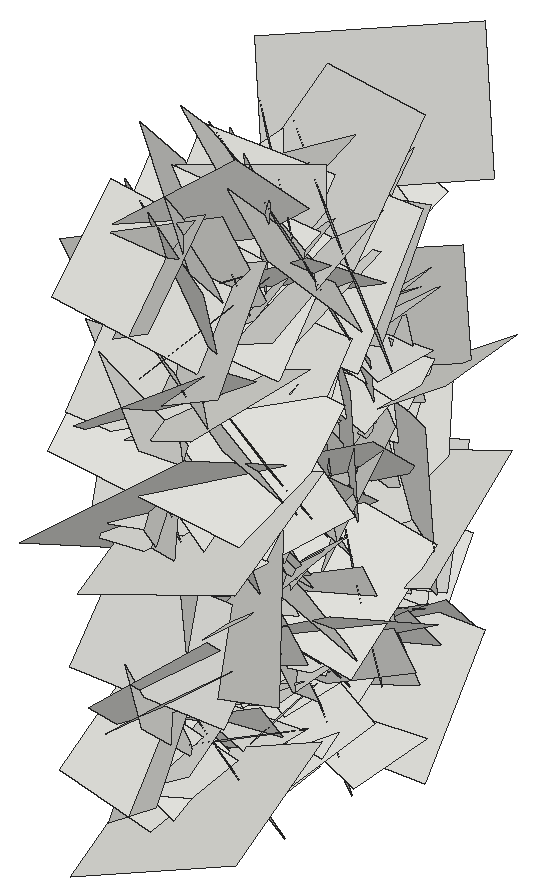
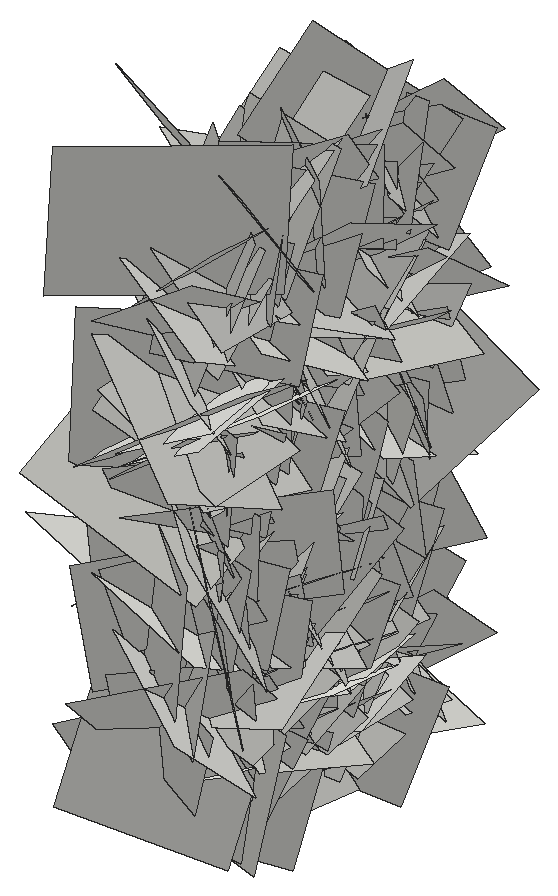
# SketchUp Ruby script. Lengths in inches.
U = 1.inch
M = Sketchup.active_model
def pt(a) = Geom::Point3d.new(a.map { |v| v * U })
def face(e, loops, mat)
  f = e.add_face(loops[0].map { |a| pt(a) })
  loops[1..].each { |l| e.add_face(l.map { |a| pt(a) }).erase! }
  f.material = f.back_material = mat if mat
  f
end
# faces: each face lists its corners as indices into pts; further lists are holes
def faces(e, pts, list, mat = nil) = list.each { |f| face(e, (f[0].is_a?(Array) ? f : [f]).map { |l| l.map { |i| pts[i] } }, mat) }
# xy, xz, yz: faces in a plane at the given z, y or x. An outline is a flat list of corners, or four numbers for a rectangle; further outlines are holes
def ring(l) = l.size == 4 ? [[l[0], l[1]], [l[2], l[1]], [l[2], l[3]], [l[0], l[3]]] : l.each_slice(2).to_a
def flat(e, list, mat, &to3) = list.each { |f| face(e, (f[0].is_a?(Array) ? f : [f]).map { |l| ring(l).map { |u, v| to3.(u, v) } }, mat) }
def xy(e, z, list, mat = nil) = flat(e, list, mat) { |x, y| [x, y, z] }
def xz(e, y, list, mat = nil) = flat(e, list, mat) { |x, z| [x, y, z] }
def yz(e, x, list, mat = nil) = flat(e, list, mat) { |y, z| [x, y, z] }
def lines(e, pts, list) = list.each { |a, b| e.add_line(pt(pts[a]), pt(pts[b])) }
# prism: a flat outline (further loops are holes) pulled along v
def prism(e, loops, v, mat = nil)
  f = face(e, loops, mat); d = Geom::Vector3d.new(v.map { |x| x * U })
  f.pushpull(f.normal.samedirection?(d) ? d.length : -d.length)
end
def box(e, o, s, mat = nil) = prism(e, [[o, [o[0] + s[0], o[1], o[2]], [o[0] + s[0], o[1] + s[1], o[2]], [o[0], o[1] + s[1], o[2]]]], [0, 0, s[2]], mat)
def at(x, y, z, deg = 0) = Geom::Transformation.translation(pt([x, y, z])) * Geom::Transformation.rotation(ORIGIN, Z_AXIS, deg.degrees)
def axes(o, x, y, z) = Geom::Transformation.new([*x, 0, *y, 0, *z, 0, *pt(o).to_a, 1])
def part(name) = M.definitions.add(name)
# library, detail: a bought-in or finely detailed component or shape, given as its bounding box
def library(name, o, s) = part(name).tap { |d| box(d.entities, o, s) }
def detail(e, o, s) = box(e.add_group.entities, o, s)
def put(e, d, t, mat = nil) = e.add_instance(d, t).tap { |i| i.material = mat if mat }
def group(e, t, mat = nil) = e.add_group.tap { |g| g.transformation = t; g.material = mat if mat }.entities
root = M.entities
c1 = part("Component\#6")
p = [[0.01,0,0],[0,3.24,4.54],[4.32,3.24,4.54],[4.33,0,0]]
faces(c1.entities,p,[[0,1,2,3]])
put(root,c1,axes([38.11,167.01,8.33],[-0.18631,0.3359,0.73427],[-0.04897,0.74605,-0.35235],[-0.8545,-0.11599,-0.1399]))
put(root,c1,axes([34.14,159.82,10.86],[-0.164,0.05549,-0.7166],[0.119,-0.72215,-0.08015],[0.75252,0.12629,-0.14349]))
put(root,c1,axes([38.11,164.72,6.23],[0.02586,0.29335,1.1723],[0.23754,1.1511,-0.29271],[-1.25874,0.22326,-0.03115]))
put(root,c1,axes([34.14,164.71,11.17],[-0.09162,-0.23701,0.75882],[-0.09076,0.76162,0.22813],[0.83777,0.05659,0.1077]))
put(root,c1,axes([34.14,167.39,12.19],[-0.06725,0.11282,-0.6237],[0.12717,-0.61335,-0.12315],[0.65971,0.12973,-0.03984]))
put(root,c1,axes([34.14,158.25,7.85],[0.01053,0.60228,-0.51533],[-0.19634,-0.49934,-0.58716],[0.81696,-0.12777,-0.13447]))
put(root,c1,axes([38.11,165.51,17.74],[-0.00528,-0.97827,-0.44464],[0.11526,-0.44282,0.97306],[-1.13321,-0.04048,0.10104]))
put(root,c1,axes([38.11,165.75,-1.09],[0.03685,-0.4153,0.96157],[0.02645,0.96216,0.41465],[-1.10996,0.00914,0.04181]))
put(root,c1,axes([38.11,167.74,3.51],[0.11337,-0.86322,0.3774],[-0.28126,0.33685,0.84566],[-0.95821,-0.201,-0.20357]))
put(root,c1,axes([38.11,161.03,4.22],[-0.00206,0.54706,-0.73945],[-0.10036,-0.73565,-0.544],[-0.96983,0.07497,0.05787]))
put(root,c1,axes([38.11,158.84,13.7],[-0.15038,-0.75335,0.50607],[0.08727,0.49942,0.76653],[-0.95804,0.16374,-0.00961]))
put(root,c1,axes([38.11,166.72,20.27],[-0.14718,0.45385,-0.66356],[-0.05291,-0.67695,-0.45256],[-0.85051,-0.03642,0.14299]))
put(root,c1,axes([34.14,158.82,19.64],[0.09205,0.73549,-0.019],[-0.17536,0.00088,-0.72213],[0.75991,-0.08889,-0.16434]))
put(root,c1,axes([38.11,169.09,13.37],[-0.12805,-0.81492,0.2825],[0.01832,0.28292,0.8235],[-0.91406,0.11983,-0.02307]))
put(root,c1,axes([34.14,159.61,12.59],[0.0897,0.16152,-0.57424],[0.01993,-0.58042,-0.16049],[0.632,-0.00462,0.08656]))
put(root,c1,axes([34.14,160.65,18.69],[0.1336,-0.1743,0.59472],[-0.06624,0.60023,0.18916],[0.65357,0.09646,-0.1024]))
put(root,c1,axes([34.14,160.54,14.42],[-0.065,-0.29459,-0.75204],[-0.0763,-0.74921,0.29935],[0.85274,-0.0895,-0.03054]))
put(root,c1,axes([34.14,161.26,10.83],[-0.08958,0.45503,-0.59155],[0.06652,-0.58889,-0.46195],[0.78829,0.10141,-0.02824]))
put(root,c1,axes([38.11,170.16,13.55],[0.14984,-1.04824,-0.22204],[-0.00627,-0.22472,1.05715],[-1.13577,-0.13705,-0.03513]))
put(root,c1,axes([34.14,160.97,6.7],[0.04912,0.73058,0.10133],[-0.09877,0.10652,-0.72536],[0.77557,-0.03271,-0.0988]))
put(root,c1,axes([38.11,163.26,10.51],[-0.09772,0.8385,-0.3881],[0.10419,-0.37892,-0.842],[-0.97385,-0.12468,-0.05114]))
put(root,c1,axes([34.14,159.79,25.07],[-0.1328,0.69586,-0.68383],[-0.18687,-0.69425,-0.67416],[1.01714,-0.03669,-0.21313]))
put(root,c1,axes([38.11,167.39,3.05],[0.22625,-1.02118,-0.283],[-0.12014,-0.30902,1.02962],[-1.11681,-0.17363,-0.16809]))
put(root,c1,axes([34.14,159.32,12.84],[0.06752,-0.16321,-0.59207],[0.0871,-0.58763,0.17083],[0.64514,0.09641,0.0389]))
put(root,c1,axes([34.14,169.73,5.36],[0.07377,0.11031,-0.61615],[0.06228,-0.61836,-0.10407],[0.66058,0.04598,0.07863]))
put(root,c1,axes([38.11,166.22,16.78],[0.0558,0.90138,-0.08554],[-0.09664,-0.07998,-0.89882],[-0.95488,0.06076,0.08597]))
put(root,c1,axes([34.14,166.8,6.58],[-0.19077,-0.84984,-0.315],[0.00737,-0.32244,0.86593],[0.9607,-0.16629,-0.0692]))
put(root,c1,axes([38.11,159.03,23.29],[0.13252,0.38295,-0.87838],[-0.10893,-0.87536,-0.39626],[-1.00987,0.14467,-0.07253]))
put(root,c1,axes([34.14,160.57,3.12],[0.03509,0.82869,0.13415],[-0.15764,0.13792,-0.81528],[0.87577,-0.00838,-0.15213]))
put(root,c1,axes([34.14,164.04,15.7],[0.03624,-0.6234,-0.24842],[0.08,-0.24359,0.62167],[0.70683,0.05954,-0.05762]))
put(root,c1,axes([38.11,170.98,12.21],[0.31631,-0.51758,-1.19288],[0.16648,-1.20059,0.56021],[-1.36826,-0.26573,-0.20761]))
put(root,c1,axes([34.14,169.83,13.22],[0.13817,-0.64015,-0.16037],[-0.03989,-0.17041,0.64965],[0.69839,0.11692,0.06883]))
put(root,c1,axes([34.14,161.46,7.67],[0.11157,-0.00104,0.59962],[0.09459,0.60203,-0.01462],[0.62852,-0.09042,-0.10424]))
put(root,c1,axes([38.11,168.08,9.41],[0.11593,0.02752,-0.90523],[-0.14705,-0.90054,-0.04413],[-0.94866,0.14295,-0.10378]))
put(root,c1,axes([34.14,169.26,18.83],[0.02849,-0.83115,-0.05333],[-0.13283,-0.05679,0.82186],[0.87278,0.01849,0.12683]))
put(root,c1,axes([34.14,165.55,15.88],[-0.02597,-0.35934,-0.67832],[0.02345,-0.67872,0.35875],[0.81334,0.00809,-0.032]))
put(root,c1,axes([34.14,167.12,21.5],[0.0656,0.35319,-0.61189],[0.00255,-0.61434,-0.35436],[0.7489,-0.02885,0.0548]))
put(root,c1,axes([38.11,164.04,2.37],[0.08884,-0.86849,0.07962],[-0.14736,0.06566,0.86256],[-0.91264,-0.09515,-0.13152]))
put(root,c1,axes([38.11,162.54,0.74],[0.05881,-0.79857,0.25436],[-0.14334,0.24305,0.79255],[-0.87675,-0.0933,-0.11251]))
put(root,c1,axes([38.11,157.37,3.29],[-0.12325,0.67494,0.21472],[-0.06797,0.20667,-0.68436],[-0.74769,-0.13004,0.02682]))
put(root,c1,axes([38.11,166.02,4.84],[0.16866,0.71959,0.68076],[-0.0323,0.69272,-0.72511],[-1.04952,0.09433,0.13172]))
put(root,c1,axes([34.14,162.4,12.14],[0.15913,-0.1111,0.71617],[-0.10617,0.72117,0.13287],[0.76084,0.12387,-0.13124]))
put(root,c1,axes([34.14,165.06,16.01],[-0.24936,0.99659,0.4051],[-0.07669,0.39908,-1.02378],[1.13774,0.24532,0.01978]))
put(root,c1,axes([34.14,164.7,6.68],[-0.19863,-0.78204,0.62344],[-0.03401,0.63866,0.7915],[1.0596,-0.1261,0.14227]))
put(root,c1,axes([38.11,166.67,11.65],[-0.03639,0.32382,0.70516],[-0.0632,0.70266,-0.32558],[-0.82009,-0.06852,-0.0062]))
put(root,c1,axes([38.11,166.25,3.34],[-0.10377,-0.78092,-0.09398],[0.04515,-0.09983,0.78516],[-0.83253,0.09192,0.05429]))
put(root,c1,axes([38.11,167.84,10.46],[0.01526,0.23241,-0.73689],[-0.14958,-0.72384,-0.23105],[-0.80526,0.13886,0.02896]))
put(root,c1,axes([38.11,164.66,7.18],[0.03191,0.54978,-0.59147],[-0.106,-0.58478,-0.54866],[-0.84939,0.09364,0.04625]))
put(root,c1,axes([38.11,155.24,20.59],[-0.01301,0.69003,0.71111],[0.211,0.69839,-0.67424],[-1.02891,0.13449,-0.14726]))
put(root,c1,axes([38.11,167.39,19.82],[-0.12929,0.6108,0.35138],[-0.02449,0.35295,-0.62154],[-0.74654,-0.11736,-0.04046]))
put(root,c1,axes([34.14,165.07,9.38],[0.13081,0.27606,-0.70722],[-0.08788,-0.70731,-0.29057],[0.79993,-0.12284,0.08373]))
put(root,c1,axes([38.11,159.79,6],[0.13547,0.51146,0.93772],[0.15367,0.92736,-0.52557],[-1.12174,0.18881,0.04125]))
put(root,c1,axes([38.11,159.9,13.67],[0.02397,0.44215,0.82689],[0.11898,0.8199,-0.44149],[-0.98679,0.1096,-0.03314]))
put(root,c1,axes([34.14,164.44,22.83],[-0.02931,-0.02413,-0.88007],[-0.04764,-0.87932,0.02552],[0.93201,-0.0457,-0.02637]))
put(root,c1,axes([38.11,168.54,15.47],[0.051,0.16682,-0.79913],[-0.09039,-0.79511,-0.17112],[-0.86061,0.0934,-0.02938]))
put(root,c1,axes([38.11,155.625,2.89],[-0.13104,0.56412,0.5606],[0.11872,0.57403,-0.55293],[-0.83462,-0.00692,-0.16667]))
put(root,c1,axes([38.11,163.43,17.5],[0.07736,-0.30856,0.98844],[0.18729,0.98007,0.2929],[-1.08152,0.14765,0.12143]))
put(root,c1,axes([34.14,163.43,17.5],[-0.07736,-0.30856,0.98844],[-0.18729,0.98007,0.2929],[1.08152,0.14765,0.12143]))
put(root,c1,axes([34.14,155.625,2.89],[0.13104,0.56412,0.5606],[-0.11872,0.57403,-0.55293],[0.83462,-0.00692,-0.16667]))
put(root,c1,axes([34.14,168.54,15.47],[-0.051,0.16682,-0.79913],[0.09039,-0.79511,-0.17112],[0.86061,0.0934,-0.02938]))
put(root,c1,axes([38.11,164.44,22.83],[0.02931,-0.02413,-0.88007],[0.04764,-0.87932,0.02552],[-0.93201,-0.0457,-0.02637]))
put(root,c1,axes([34.14,159.9,13.67],[-0.02397,0.44215,0.82689],[-0.11898,0.8199,-0.44149],[0.98679,0.1096,-0.03314]))
put(root,c1,axes([34.14,159.79,6],[-0.13547,0.51146,0.93772],[-0.15367,0.92736,-0.52557],[1.12174,0.18881,0.04125]))
put(root,c1,axes([38.11,165.07,9.38],[-0.13081,0.27606,-0.70722],[0.08788,-0.70731,-0.29057],[-0.79993,-0.12284,0.08373]))
put(root,c1,axes([34.14,167.39,19.82],[0.12929,0.6108,0.35138],[0.02449,0.35295,-0.62154],[0.74654,-0.11736,-0.04046]))
put(root,c1,axes([34.14,155.24,20.59],[0.01301,0.69003,0.71111],[-0.211,0.69839,-0.67424],[1.02891,0.13449,-0.14726]))
put(root,c1,axes([34.14,164.66,7.18],[-0.03191,0.54978,-0.59147],[0.106,-0.58478,-0.54866],[0.84939,0.09364,0.04625]))
put(root,c1,axes([34.14,167.84,10.46],[-0.01526,0.23241,-0.73689],[0.14958,-0.72384,-0.23105],[0.80526,0.13886,0.02896]))
put(root,c1,axes([34.14,166.25,3.34],[0.10377,-0.78092,-0.09398],[-0.04515,-0.09983,0.78516],[0.83253,0.09192,0.05429]))
put(root,c1,axes([34.14,166.67,11.65],[0.03639,0.32382,0.70516],[0.0632,0.70266,-0.32558],[0.82009,-0.06852,-0.0062]))
put(root,c1,axes([38.11,164.7,6.68],[0.19863,-0.78204,0.62344],[0.03401,0.63866,0.7915],[-1.0596,-0.1261,0.14227]))
put(root,c1,axes([38.11,165.06,16.01],[0.24936,0.99659,0.4051],[0.07669,0.39908,-1.02378],[-1.13774,0.24532,0.01978]))
put(root,c1,axes([38.11,162.4,12.14],[-0.15913,-0.1111,0.71617],[0.10617,0.72117,0.13287],[-0.76084,0.12387,-0.13124]))
put(root,c1,axes([34.14,166.02,4.84],[-0.16866,0.71959,0.68076],[0.0323,0.69272,-0.72511],[1.04952,0.09433,0.13172]))
put(root,c1,axes([34.14,157.37,3.29],[0.12325,0.67494,0.21472],[0.06797,0.20667,-0.68436],[0.74769,-0.13004,0.02682]))
put(root,c1,axes([34.14,162.54,0.74],[-0.05881,-0.79857,0.25436],[0.14334,0.24305,0.79255],[0.87675,-0.0933,-0.11251]))
put(root,c1,axes([34.14,164.04,2.37],[-0.08884,-0.86849,0.07962],[0.14736,0.06566,0.86256],[0.91264,-0.09515,-0.13152]))
put(root,c1,axes([38.11,167.12,21.5],[-0.0656,0.35319,-0.61189],[-0.00255,-0.61434,-0.35436],[-0.7489,-0.02885,0.0548]))
put(root,c1,axes([38.11,165.55,15.88],[0.02597,-0.35934,-0.67832],[-0.02345,-0.67872,0.35875],[-0.81334,0.00809,-0.032]))
put(root,c1,axes([38.11,169.26,18.83],[-0.02849,-0.83115,-0.05333],[0.13283,-0.05679,0.82186],[-0.87278,0.01849,0.12683]))
put(root,c1,axes([34.14,168.08,9.41],[-0.11593,0.02752,-0.90523],[0.14705,-0.90054,-0.04413],[0.94866,0.14295,-0.10378]))
put(root,c1,axes([38.11,161.46,7.67],[-0.11157,-0.00104,0.59962],[-0.09459,0.60203,-0.01462],[-0.62852,-0.09042,-0.10424]))
put(root,c1,axes([38.11,169.83,13.22],[-0.13817,-0.64015,-0.16037],[0.03989,-0.17041,0.64965],[-0.69839,0.11692,0.06883]))
put(root,c1,axes([34.14,170.98,12.21],[-0.31631,-0.51758,-1.19288],[-0.16648,-1.20059,0.56021],[1.36826,-0.26573,-0.20761]))
put(root,c1,axes([38.11,164.04,15.7],[-0.03624,-0.6234,-0.24842],[-0.08,-0.24359,0.62167],[-0.70683,0.05954,-0.05762]))
put(root,c1,axes([38.11,160.57,3.12],[-0.03509,0.82869,0.13415],[0.15764,0.13792,-0.81528],[-0.87577,-0.00838,-0.15213]))
put(root,c1,axes([34.14,159.03,23.29],[-0.13252,0.38295,-0.87838],[0.10893,-0.87536,-0.39626],[1.00987,0.14467,-0.07253]))
put(root,c1,axes([38.11,166.8,6.58],[0.19077,-0.84984,-0.315],[-0.00737,-0.32244,0.86593],[-0.9607,-0.16629,-0.0692]))
put(root,c1,axes([34.14,166.22,16.78],[-0.0558,0.90138,-0.08554],[0.09664,-0.07998,-0.89882],[0.95488,0.06076,0.08597]))
put(root,c1,axes([38.11,159.32,12.84],[-0.06752,-0.16321,-0.59207],[-0.0871,-0.58763,0.17083],[-0.64514,0.09641,0.0389]))
put(root,c1,axes([34.14,167.39,3.05],[-0.22625,-1.02118,-0.283],[0.12014,-0.30902,1.02962],[1.11681,-0.17363,-0.16809]))
put(root,c1,axes([38.11,159.79,25.07],[0.1328,0.69586,-0.68383],[0.18687,-0.69425,-0.67416],[-1.01714,-0.03669,-0.21313]))
put(root,c1,axes([34.14,163.26,10.51],[0.09772,0.8385,-0.3881],[-0.10419,-0.37892,-0.842],[0.97385,-0.12468,-0.05114]))
put(root,c1,axes([38.11,160.97,6.7],[-0.04912,0.73058,0.10133],[0.09877,0.10652,-0.72536],[-0.77557,-0.03271,-0.0988]))
put(root,c1,axes([34.14,170.16,13.55],[-0.14984,-1.04824,-0.22204],[0.00627,-0.22472,1.05715],[1.13577,-0.13705,-0.03513]))
put(root,c1,axes([38.11,161.26,10.83],[0.08958,0.45503,-0.59155],[-0.06652,-0.58889,-0.46195],[-0.78829,0.10141,-0.02824]))
put(root,c1,axes([38.11,160.54,14.42],[0.065,-0.29459,-0.75204],[0.0763,-0.74921,0.29935],[-0.85274,-0.0895,-0.03054]))
put(root,c1,axes([38.11,160.65,18.69],[-0.1336,-0.1743,0.59472],[0.06624,0.60023,0.18916],[-0.65357,0.09646,-0.1024]))
put(root,c1,axes([38.11,159.61,12.59],[-0.0897,0.16152,-0.57424],[-0.01993,-0.58042,-0.16049],[-0.632,-0.00462,0.08656]))
put(root,c1,axes([34.14,169.09,13.37],[0.12805,-0.81492,0.2825],[-0.01832,0.28292,0.8235],[0.91406,0.11983,-0.02307]))
put(root,c1,axes([38.11,158.82,19.64],[-0.09205,0.73549,-0.019],[0.17536,0.00088,-0.72213],[-0.75991,-0.08889,-0.16434]))
put(root,c1,axes([34.14,166.72,20.27],[0.14718,0.45385,-0.66356],[0.05291,-0.67695,-0.45256],[0.85051,-0.03642,0.14299]))
put(root,c1,axes([34.14,158.84,13.7],[0.15038,-0.75335,0.50607],[-0.08727,0.49942,0.76653],[0.95804,0.16374,-0.00961]))
put(root,c1,axes([34.14,161.03,4.22],[0.00206,0.54706,-0.73945],[0.10036,-0.73565,-0.544],[0.96983,0.07497,0.05787]))
put(root,c1,axes([34.14,167.74,3.51],[-0.11337,-0.86322,0.3774],[0.28126,0.33685,0.84566],[0.95821,-0.201,-0.20357]))
put(root,c1,axes([34.14,165.75,-1.09],[-0.03685,-0.4153,0.96157],[-0.02645,0.96216,0.41465],[1.10996,0.00914,0.04181]))
put(root,c1,axes([34.14,165.51,17.74],[0.00528,-0.97827,-0.44464],[-0.11526,-0.44282,0.97306],[1.13321,-0.04048,0.10104]))
put(root,c1,axes([38.11,158.25,7.85],[-0.01053,0.60228,-0.51533],[0.19634,-0.49934,-0.58716],[-0.81696,-0.12777,-0.13447]))
put(root,c1,axes([38.11,167.39,12.19],[0.06725,0.11282,-0.6237],[-0.12717,-0.61335,-0.12315],[-0.65971,0.12973,-0.03984]))
put(root,c1,axes([38.11,164.71,11.17],[0.09162,-0.23701,0.75882],[0.09076,0.76162,0.22813],[-0.83777,0.05659,0.1077]))
put(root,c1,axes([34.14,164.72,6.23],[-0.02586,0.29335,1.1723],[-0.23754,1.1511,-0.29271],[1.25874,0.22326,-0.03115]))
put(root,c1,axes([38.11,159.82,10.86],[0.164,0.05549,-0.7166],[-0.119,-0.72215,-0.08015],[-0.75252,0.12629,-0.14349]))
put(root,c1,axes([34.14,167.01,8.33],[0.18631,0.3359,0.73427],[0.04897,0.74605,-0.35235],[0.8545,-0.11599,-0.1399]))
put(root,c1,axes([34.14,166.18,19.56],[-0.12535,0.0531,1.28965],[-0.2192,1.27754,-0.07157],[1.35051,0.21229,0.10808]))
put(root,c1,axes([34.14,168.14,0.12],[-0.06773,-0.63363,0.78179],[0.11595,0.77435,0.63654],[1.06038,-0.12515,-0.01967]))
put(root,c1,axes([34.14,169.19,10.7],[-0.0913,0.46499,-1.24639],[-0.29576,-1.22753,-0.43867],[1.37875,-0.23253,-0.17663]))
put(root,c1,axes([38.11,165.96,10.85],[0.09912,0.20412,-0.70693],[0.02587,-0.71308,-0.20267],[-0.77953,0.00229,-0.09661]))
put(root,c1,axes([38.11,161.25,17.66],[0.25985,0.898,-0.37026],[0.14737,-0.41038,-0.90325],[-1.01902,0.16964,-0.22504]))
put(root,c1,axes([38.11,162.79,15.86],[0.07285,0.46729,0.4905],[-0.02436,0.49435,-0.46773],[-0.71769,0.03066,0.06566]))
put(root,c1,axes([34.14,167.22,15.375],[-0.0235,-0.92066,-0.53568],[-0.01768,-0.53543,0.92093],[1.12894,-0.02755,0.00327]))
put(root,c1,axes([34.14,167.28,17.92],[-0.19972,-0.96368,-0.57877],[0.14667,-0.60226,0.95775],[1.18251,-0.08806,-0.21655]))
put(root,c1,axes([34.14,157.18,19.73],[-0.07599,0.81527,0.8297],[-0.084,0.82592,-0.8184],[1.23014,0.10676,-0.00463]))
put(root,c1,axes([34.14,167.18,1.59],[-0.07507,-1.0991,0.32301],[-0.05871,0.32653,1.09895],[1.2129,-0.05222,0.07319]))
put(root,c1,axes([34.14,168.87,14.79],[0.03205,0.06087,-1.12787],[-0.16204,-1.11767,-0.06442],[1.18627,-0.15431,0.02167]))
put(root,c1,axes([34.14,166.01,11.8],[0.21466,0.53877,-0.68228],[-0.03009,-0.69607,-0.55809],[0.92102,-0.14831,0.14079]))
put(root,c1,axes([34.14,163.57,3.71],[0.11292,-0.2033,0.99476],[-0.09749,0.99417,0.21302],[1.07181,0.11185,-0.08542]))
put(root,c1,axes([34.14,159.91,9.22],[-0.2022,-1.20502,0.50539],[-0.1049,0.52261,1.20871],[1.38114,-0.13672,0.1658]))
put(root,c1,axes([34.14,162.44,14.8125],[-0.22172,-1.13603,-0.19278],[0.19013,-0.22565,1.13507],[1.20652,-0.17321,-0.21429]))
put(root,c1,axes([34.14,160.62,5.12],[0.08568,1.04485,0.18773],[-0.09569,0.19436,-1.04286],[1.1212,-0.06325,-0.10335]))
put(root,c1,axes([38.11,162.91,7.6875],[0.03517,0.6334,0.29771],[0.1292,0.28826,-0.62688],[-0.73053,0.08147,-0.09654]))
put(root,c1,axes([34.14,163.93,5.47],[0.11462,-1.01834,-0.26907],[-0.10191,-0.2789,1.0169],[1.11183,0.07941,0.12095]))
put(root,c1,axes([34.14,156.14,6.5],[0.17845,0.35117,0.84391],[0.01887,0.85668,-0.36003],[0.96872,-0.08137,-0.14844]))
put(root,c1,axes([38.11,170.02,6.34],[0.13634,-0.30577,-0.6303],[0.02329,-0.63876,0.31436],[-0.74222,-0.07621,-0.10592]))
put(root,c1,axes([34.14,160.14,4.78],[0.03826,-0.47304,0.81506],[0.18962,0.80427,0.45886],[0.98077,-0.13704,-0.12051]))
put(root,c1,axes([34.14,166.625,12.7],[0.17127,1.04033,-0.10676],[-0.13463,-0.08771,-1.04688],[1.10034,-0.17266,-0.11147]))
put(root,c1,axes([34.14,168.99,0.33],[0.20008,-0.71049,0.66963],[-0.07161,0.67089,0.73087],[1.03242,0.18422,-0.07908]))
put(root,c1,axes([34.14,164.18,5.53],[0.00871,-1.21515,-0.1589],[-0.11926,-0.15898,1.20995],[1.29354,-0.00648,0.11262]))
put(root,c1,axes([38.11,159.77,13.93],[0.14822,0.47929,0.38572],[-0.01533,0.39801,-0.48932],[-0.65196,0.0996,0.0992]))
put(root,c1,axes([34.14,165.6875,8.33],[0.14254,-0.77018,0.64298],[0.05856,0.65343,0.77114],[1.06187,0.06735,-0.12884]))
put(root,c1,axes([34.14,164.53,2.65],[0.11418,0.95876,0.15487],[0.16789,0.13639,-0.95453],[1.01568,-0.13033,0.14037]))
put(root,c1,axes([38.11,155.94,6.59],[0.14653,0.65267,0.04592],[0.0729,0.03218,-0.6644],[-0.6897,0.14207,-0.06047]))
put(root,c1,axes([34.14,170.79,17.67],[0.07972,-0.69903,-0.88266],[-0.01234,-0.88506,0.69994],[1.19343,0.03754,0.0662]))
put(root,c1,axes([34.14,165.97,13.03],[0.11695,-0.23373,1.15092],[-0.10796,1.14973,0.24325],[1.24018,0.12213,-0.08736]))
put(root,c1,axes([38.11,164.09,3.1],[0.16189,-0.51758,0.36968],[0.06161,0.38995,0.52196],[-0.67139,-0.08902,0.13704]))
put(root,c1,axes([34.14,155.93,16.01],[0.06166,0.77521,1.08886],[-0.24821,1.07895,-0.75564],[1.39492,0.15772,-0.18259]))
put(root,c1,axes([34.14,163.21,2.24],[-0.08398,-0.53221,1.10764],[0.11648,1.10243,0.53756],[1.29738,-0.13342,0.02343]))
put(root,c1,axes([34.14,161.02,12.77],[0.04866,0.36936,-1.04237],[0.12613,-1.03886,-0.36288],[1.16543,0.09701,0.0828]))
put(root,c1,axes([34.14,162.03,18.62],[0.15865,-0.78055,-0.79386],[-0.03617,-0.80384,0.78393],[1.17956,0.08034,0.13081]))
put(root,c1,axes([34.14,161.03,16.77],[-0.02327,0.73455,-0.90907],[0.17416,-0.89826,-0.72978],[1.22657,0.14148,0.08637]))
put(root,c1,axes([34.14,163.86,1.73],[0.03729,0.66749,1.03354],[-0.00972,1.03407,-0.66752],[1.30413,-0.01138,-0.03452]))
put(root,c1,axes([34.14,162.85,15.75],[0.04254,-1.00522,0.67204],[0.02385,0.67292,1.00519],[1.28151,0.02084,-0.04102]))
put(root,c1,axes([34.14,163.36,23.49],[0.04873,0.57368,-1.00395],[0.12423,-1.00188,-0.56714],[1.21936,0.07915,0.09791]))
put(root,c1,axes([34.14,159.69,18.96],[0.02704,0.74145,1.09535],[-0.09362,1.09406,-0.73853],[1.39894,0.05888,-0.07059]))
put(root,c1,axes([34.14,166.4,18.65],[-0.092,-1.19571,-0.63762],[0.0325,-0.6405,1.19693],[1.43603,-0.06211,-0.06794]))
put(root,c1,axes([34.14,155.03,14.95],[-0.10989,1.07322,0.82249],[0.07177,0.82799,-1.07186],[1.43147,0.04087,0.11688]))
put(root,c1,axes([34.14,159.14,18.38],[0.07521,0.79304,-0.86536],[0.12573,-0.86735,-0.78513],[1.23784,0.03991,0.13233]))
put(root,c1,axes([34.14,168.375,23.9],[-0.0952,-0.72561,-1.04974],[0.29336,-1.03837,0.69407],[1.32049,0.17837,-0.22987]))
put(root,c1,axes([34.14,157.93,15.34],[0.27083,1.19165,0.15594],[-0.0802,0.17506,-1.21378],[1.27139,-0.2428,-0.10978]))
put(root,c1,axes([34.14,162.31,11.53],[0.17206,0.75955,-0.87532],[0.12131,-0.89005,-0.75111],[1.22246,-0.01858,0.19774]))
put(root,c1,axes([34.14,165.1,2.71],[-0.06092,-1.21711,0.58199],[0.18306,0.57109,1.21136],[1.41828,-0.12599,-0.13136]))
put(root,c1,axes([34.14,170.58,10.37],[0.24309,-1.14649,0.14454],[0.04952,0.15643,1.16674],[1.2239,0.22139,-0.07591]))
put(root,c1,axes([34.14,161.07,7.88],[0.0926,0.91308,0.78861],[0.24837,0.76278,-0.90913],[1.25453,-0.21841,0.12178]))
put(root,c1,axes([34.14,171.01,11.29],[0.23144,-0.15428,-1.27652],[-0.01824,-1.29503,0.15357],[1.36284,0.00887,0.21884]))
put(root,c1,axes([34.14,167.61,21.95],[0.32344,0.31012,-1.26322],[-0.1451,-1.28265,-0.34796],[1.37111,-0.2089,0.26116]))
put(root,c1,axes([34.14,161.91,24.73],[0.20116,0.87735,-0.9177],[0.06395,-0.93308,-0.87958],[1.34427,-0.0869,0.17917]))
put(root,c1,axes([34.14,161.24,11.55],[0.08722,-1.18104,-0.51149],[0.30261,-0.48302,1.16122],[1.33028,0.18731,-0.23062]))
put(root,c1,axes([34.14,160.65,1.35],[0.1594,-1.22011,-0.46707],[0.28659,-0.43091,1.2127],[1.35486,0.2347,-0.20157]))
put(root,c1,axes([34.14,170.67,8.29],[0.13658,-1.14766,-0.62909],[0.33753,-0.58565,1.13362],[1.34561,0.26339,-0.2205]))
put(root,c1,axes([34.14,161.87,9.58],[0.35888,-0.49511,-1.17449],[0.11741,-1.19919,0.53746],[1.34594,0.23663,0.26628]))
